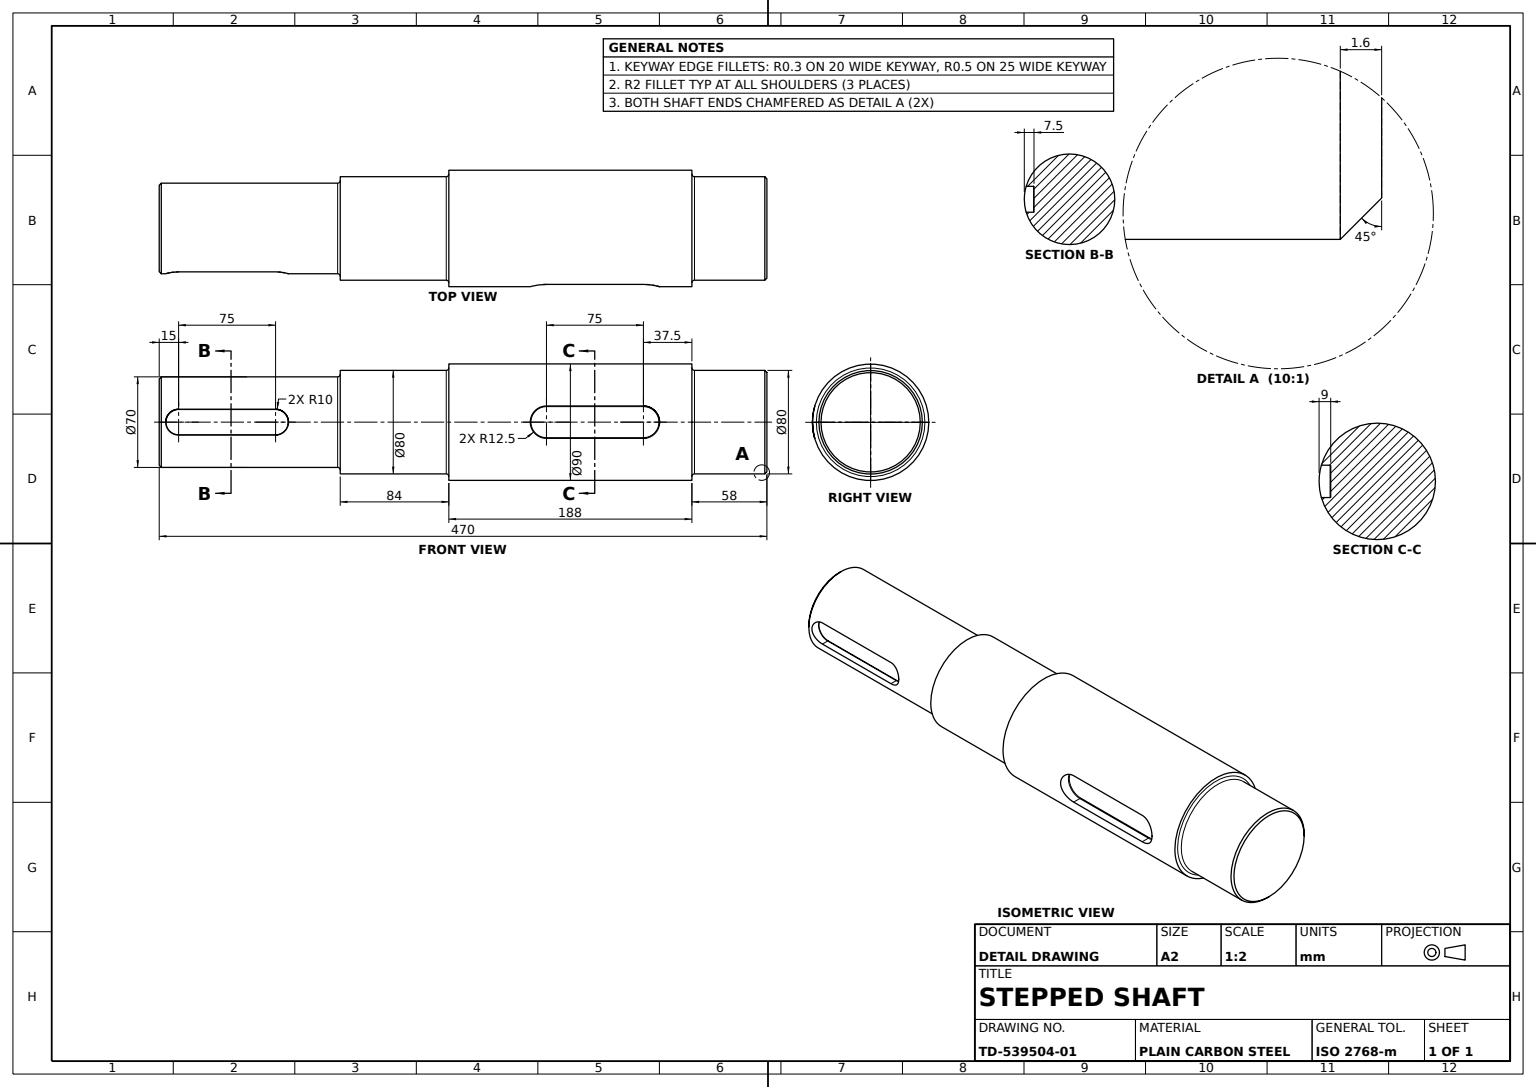
ISO-10303-21;
HEADER;
FILE_DESCRIPTION((''),'2;1');
FILE_NAME('','',(''),(''),'','','');
FILE_SCHEMA(('AUTOMOTIVE_DESIGN'));
ENDSEC;
DATA;
#1=APPLICATION_CONTEXT('');
#2=PRODUCT_CONTEXT('',#1,'mechanical');
#3=PRODUCT('','','',(#2));
#4=PRODUCT_DEFINITION_FORMATION('','',#3);
#5=PRODUCT_DEFINITION_CONTEXT('',#1,'design');
#6=PRODUCT_DEFINITION('','',#4,#5);
#7=PRODUCT_DEFINITION_SHAPE('','',#6);
#8=(LENGTH_UNIT()NAMED_UNIT(*)SI_UNIT(.MILLI.,.METRE.));
#9=(NAMED_UNIT(*)PLANE_ANGLE_UNIT()SI_UNIT($,.RADIAN.));
#10=(NAMED_UNIT(*)SI_UNIT($,.STERADIAN.)SOLID_ANGLE_UNIT());
#11=UNCERTAINTY_MEASURE_WITH_UNIT(LENGTH_MEASURE(1.E-05),#8,'distance_accuracy_value','');
#12=(GEOMETRIC_REPRESENTATION_CONTEXT(3)GLOBAL_UNCERTAINTY_ASSIGNED_CONTEXT((#11))GLOBAL_UNIT_ASSIGNED_CONTEXT((#8,#9,#10))REPRESENTATION_CONTEXT('',''));
#13=CARTESIAN_POINT('',(27.8,-10.,134.));
#14=VERTEX_POINT('',#13);
#15=CARTESIAN_POINT('',(27.5,-9.7,134.));
#16=VERTEX_POINT('',#15);
#17=CARTESIAN_POINT('',(27.8,-9.7,134.));
#18=DIRECTION('',(0.,0.,-1.));
#19=DIRECTION('',(-1.,0.,0.));
#20=AXIS2_PLACEMENT_3D('',#17,#18,#19);
#21=CIRCLE('',#20,0.3);
#22=EDGE_CURVE('',#14,#16,#21,.T.);
#23=ORIENTED_EDGE('',*,*,#22,.F.);
#24=CARTESIAN_POINT('',(27.8,0.,124.));
#25=VERTEX_POINT('',#24);
#26=CARTESIAN_POINT('',(27.8,0.,134.));
#27=AXIS2_PLACEMENT_3D('',#26,#19,#18);
#28=CIRCLE('',#27,10.);
#29=EDGE_CURVE('',#25,#14,#28,.T.);
#30=ORIENTED_EDGE('',*,*,#29,.F.);
#31=CARTESIAN_POINT('',(27.5,0.,124.3));
#32=VERTEX_POINT('',#31);
#33=CARTESIAN_POINT('',(27.8,0.,124.3));
#34=DIRECTION('',(0.,-1.,0.));
#35=AXIS2_PLACEMENT_3D('',#33,#34,#18);
#36=CIRCLE('',#35,0.3);
#37=EDGE_CURVE('',#32,#25,#36,.T.);
#38=ORIENTED_EDGE('',*,*,#37,.F.);
#39=CARTESIAN_POINT('',(27.5,0.,134.));
#40=DIRECTION('',(1.,0.,0.));
#41=AXIS2_PLACEMENT_3D('',#39,#40,#18);
#42=CIRCLE('',#41,9.7);
#43=EDGE_CURVE('',#16,#32,#42,.T.);
#44=ORIENTED_EDGE('',*,*,#43,.F.);
#45=EDGE_LOOP('',(#23,#30,#38,#44));
#46=FACE_OUTER_BOUND('',#45,.T.);
#47=AXIS2_PLACEMENT_3D('',#26,#40,#18);
#48=TOROIDAL_SURFACE('',#47,9.7,0.3);
#49=ADVANCED_FACE('',(#46),#48,.F.);
#50=CARTESIAN_POINT('',(40.,0.,84.));
#51=VERTEX_POINT('',#50);
#52=CARTESIAN_POINT('',(-40.,0.,84.));
#53=VERTEX_POINT('',#52);
#54=CARTESIAN_POINT('',(0.,0.,84.));
#55=DIRECTION('',(0.,0.,1.));
#56=AXIS2_PLACEMENT_3D('',#54,#55,#40);
#57=CIRCLE('',#56,40.);
#58=EDGE_CURVE('',#51,#53,#57,.T.);
#59=ORIENTED_EDGE('',*,*,#58,.T.);
#60=EDGE_CURVE('',#53,#51,#57,.T.);
#61=ORIENTED_EDGE('',*,*,#60,.T.);
#62=EDGE_LOOP('',(#59,#61));
#63=FACE_OUTER_BOUND('',#62,.T.);
#64=CARTESIAN_POINT('',(37.,0.,84.));
#65=VERTEX_POINT('',#64);
#66=CARTESIAN_POINT('',(-37.,0.,84.));
#67=VERTEX_POINT('',#66);
#68=AXIS2_PLACEMENT_3D('',#54,#18,#40);
#69=CIRCLE('',#68,37.);
#70=EDGE_CURVE('',#65,#67,#69,.T.);
#71=ORIENTED_EDGE('',*,*,#70,.T.);
#72=EDGE_CURVE('',#67,#65,#69,.T.);
#73=ORIENTED_EDGE('',*,*,#72,.T.);
#74=EDGE_LOOP('',(#71,#73));
#75=FACE_BOUND('',#74,.T.);
#76=CARTESIAN_POINT('',(0.,-35.,84.));
#77=AXIS2_PLACEMENT_3D('',#76,#55,#40);
#78=PLANE('',#77);
#79=ADVANCED_FACE('',(#63,#75),#78,.T.);
#80=CARTESIAN_POINT('',(36.,-12.,-75.5));
#81=VERTEX_POINT('',#80);
#82=CARTESIAN_POINT('',(36.5,-12.5,-75.5));
#83=VERTEX_POINT('',#82);
#84=CARTESIAN_POINT('',(36.5,-12.,-75.5));
#85=AXIS2_PLACEMENT_3D('',#84,#55,#40);
#86=CIRCLE('',#85,0.5);
#87=EDGE_CURVE('',#81,#83,#86,.T.);
#88=ORIENTED_EDGE('',*,*,#87,.F.);
#89=CARTESIAN_POINT('',(36.,12.,-75.5));
#90=VERTEX_POINT('',#89);
#91=CARTESIAN_POINT('',(36.,0.,-75.5));
#92=AXIS2_PLACEMENT_3D('',#91,#40,#18);
#93=CIRCLE('',#92,12.);
#94=EDGE_CURVE('',#90,#81,#93,.T.);
#95=ORIENTED_EDGE('',*,*,#94,.F.);
#96=CARTESIAN_POINT('',(36.5,12.5,-75.5));
#97=VERTEX_POINT('',#96);
#98=CARTESIAN_POINT('',(36.5,12.,-75.5));
#99=AXIS2_PLACEMENT_3D('',#98,#55,#40);
#100=CIRCLE('',#99,0.5);
#101=EDGE_CURVE('',#97,#90,#100,.T.);
#102=ORIENTED_EDGE('',*,*,#101,.F.);
#103=CARTESIAN_POINT('',(36.5,0.,-75.5));
#104=AXIS2_PLACEMENT_3D('',#103,#19,#18);
#105=CIRCLE('',#104,12.5);
#106=EDGE_CURVE('',#83,#97,#105,.T.);
#107=ORIENTED_EDGE('',*,*,#106,.F.);
#108=EDGE_LOOP('',(#88,#95,#102,#107));
#109=FACE_OUTER_BOUND('',#108,.T.);
#110=AXIS2_PLACEMENT_3D('',#103,#40,#18);
#111=TOROIDAL_SURFACE('',#110,12.,0.5);
#112=ADVANCED_FACE('',(#109),#111,.F.);
#113=CARTESIAN_POINT('',(40.,0.,-244.4));
#114=VERTEX_POINT('',#113);
#115=CARTESIAN_POINT('',(40.,0.,-190.));
#116=VERTEX_POINT('',#115);
#117=CARTESIAN_POINT('',(40.,0.,224.));
#118=VECTOR('',#55,1000.);
#119=LINE('',#117,#118);
#120=EDGE_CURVE('',#114,#116,#119,.T.);
#121=ORIENTED_EDGE('',*,*,#120,.T.);
#122=CARTESIAN_POINT('',(-40.,0.,-190.));
#123=VERTEX_POINT('',#122);
#124=CARTESIAN_POINT('',(0.,0.,-190.));
#125=AXIS2_PLACEMENT_3D('',#124,#18,#19);
#126=CIRCLE('',#125,40.);
#127=EDGE_CURVE('',#116,#123,#126,.T.);
#128=ORIENTED_EDGE('',*,*,#127,.T.);
#129=CARTESIAN_POINT('',(-40.,0.,-244.4));
#130=VERTEX_POINT('',#129);
#131=CARTESIAN_POINT('',(-40.,0.,224.));
#132=LINE('',#131,#118);
#133=EDGE_CURVE('',#130,#123,#132,.T.);
#134=ORIENTED_EDGE('',*,*,#133,.F.);
#135=CARTESIAN_POINT('',(0.,0.,-244.4));
#136=AXIS2_PLACEMENT_3D('',#135,#55,#19);
#137=CIRCLE('',#136,40.);
#138=EDGE_CURVE('',#130,#114,#137,.T.);
#139=ORIENTED_EDGE('',*,*,#138,.T.);
#140=EDGE_LOOP('',(#121,#128,#134,#139));
#141=FACE_OUTER_BOUND('',#140,.T.);
#142=CARTESIAN_POINT('',(0.,0.,224.));
#143=AXIS2_PLACEMENT_3D('',#142,#55,#40);
#144=CYLINDRICAL_SURFACE('',#143,40.);
#145=ADVANCED_FACE('',(#141),#144,.T.);
#146=CARTESIAN_POINT('',(27.5,9.7,209.));
#147=VERTEX_POINT('',#146);
#148=CARTESIAN_POINT('',(27.8,10.,209.));
#149=VERTEX_POINT('',#148);
#150=CARTESIAN_POINT('',(27.8,9.7,209.));
#151=AXIS2_PLACEMENT_3D('',#150,#18,#19);
#152=CIRCLE('',#151,0.3);
#153=EDGE_CURVE('',#147,#149,#152,.T.);
#154=ORIENTED_EDGE('',*,*,#153,.T.);
#155=CARTESIAN_POINT('',(27.8,-10.,209.));
#156=VERTEX_POINT('',#155);
#157=CARTESIAN_POINT('',(27.8,0.,209.));
#158=AXIS2_PLACEMENT_3D('',#157,#19,#18);
#159=CIRCLE('',#158,10.);
#160=EDGE_CURVE('',#156,#149,#159,.T.);
#161=ORIENTED_EDGE('',*,*,#160,.F.);
#162=CARTESIAN_POINT('',(27.5,-9.7,209.));
#163=VERTEX_POINT('',#162);
#164=CARTESIAN_POINT('',(27.8,-9.7,209.));
#165=AXIS2_PLACEMENT_3D('',#164,#55,#40);
#166=CIRCLE('',#165,0.3);
#167=EDGE_CURVE('',#163,#156,#166,.T.);
#168=ORIENTED_EDGE('',*,*,#167,.F.);
#169=CARTESIAN_POINT('',(27.5,0.,209.));
#170=AXIS2_PLACEMENT_3D('',#169,#40,#18);
#171=CIRCLE('',#170,9.7);
#172=EDGE_CURVE('',#147,#163,#171,.T.);
#173=ORIENTED_EDGE('',*,*,#172,.F.);
#174=EDGE_LOOP('',(#154,#161,#168,#173));
#175=FACE_OUTER_BOUND('',#174,.T.);
#176=AXIS2_PLACEMENT_3D('',#157,#40,#18);
#177=TOROIDAL_SURFACE('',#176,9.7,0.3);
#178=ADVANCED_FACE('',(#175),#177,.F.);
#179=CARTESIAN_POINT('',(38.4,0.,-246.));
#180=VERTEX_POINT('',#179);
#181=CARTESIAN_POINT('',(-38.4,0.,-246.));
#182=VERTEX_POINT('',#181);
#183=CARTESIAN_POINT('',(0.,0.,-246.));
#184=AXIS2_PLACEMENT_3D('',#183,#18,#19);
#185=CIRCLE('',#184,38.4);
#186=EDGE_CURVE('',#180,#182,#185,.T.);
#187=ORIENTED_EDGE('',*,*,#186,.F.);
#188=DIRECTION('',(0.707106781,0.,0.707106781));
#189=VECTOR('',#188,1000.);
#190=LINE('',#113,#189);
#191=EDGE_CURVE('',#180,#114,#190,.T.);
#192=ORIENTED_EDGE('',*,*,#191,.T.);
#193=ORIENTED_EDGE('',*,*,#138,.F.);
#194=DIRECTION('',(-0.707106781,0.,0.707106781));
#195=VECTOR('',#194,1000.);
#196=LINE('',#129,#195);
#197=EDGE_CURVE('',#182,#130,#196,.T.);
#198=ORIENTED_EDGE('',*,*,#197,.F.);
#199=EDGE_LOOP('',(#187,#192,#193,#198));
#200=FACE_OUTER_BOUND('',#199,.T.);
#201=AXIS2_PLACEMENT_3D('',#135,#55,#40);
#202=CONICAL_SURFACE('',#201,40.,0.785398163);
#203=ADVANCED_FACE('',(#200),#202,.T.);
#204=CARTESIAN_POINT('',(42.,0.,0.));
#205=VERTEX_POINT('',#204);
#206=CARTESIAN_POINT('',(-42.,0.,0.));
#207=VERTEX_POINT('',#206);
#208=CARTESIAN_POINT('',(0.,0.,0.));
#209=AXIS2_PLACEMENT_3D('',#208,#18,#40);
#210=CIRCLE('',#209,42.);
#211=EDGE_CURVE('',#205,#207,#210,.T.);
#212=ORIENTED_EDGE('',*,*,#211,.F.);
#213=CARTESIAN_POINT('',(40.,0.,2.));
#214=VERTEX_POINT('',#213);
#215=CARTESIAN_POINT('',(42.,0.,2.));
#216=AXIS2_PLACEMENT_3D('',#215,#34,#18);
#217=CIRCLE('',#216,2.);
#218=EDGE_CURVE('',#214,#205,#217,.T.);
#219=ORIENTED_EDGE('',*,*,#218,.F.);
#220=CARTESIAN_POINT('',(-40.,0.,2.));
#221=VERTEX_POINT('',#220);
#222=CARTESIAN_POINT('',(0.,0.,2.));
#223=AXIS2_PLACEMENT_3D('',#222,#55,#40);
#224=CIRCLE('',#223,40.);
#225=EDGE_CURVE('',#221,#214,#224,.T.);
#226=ORIENTED_EDGE('',*,*,#225,.F.);
#227=CARTESIAN_POINT('',(-42.,0.,2.));
#228=DIRECTION('',(0.,1.,0.));
#229=AXIS2_PLACEMENT_3D('',#227,#228,#19);
#230=CIRCLE('',#229,2.);
#231=EDGE_CURVE('',#221,#207,#230,.T.);
#232=ORIENTED_EDGE('',*,*,#231,.T.);
#233=EDGE_LOOP('',(#212,#219,#226,#232));
#234=FACE_OUTER_BOUND('',#233,.T.);
#235=TOROIDAL_SURFACE('',#223,42.,2.);
#236=ADVANCED_FACE('',(#234),#235,.F.);
#237=CARTESIAN_POINT('',(43.229041,12.5,-75.5));
#238=VERTEX_POINT('',#237);
#239=CARTESIAN_POINT('',(45.,0.,-63.));
#240=VERTEX_POINT('',#239);
#241=CARTESIAN_POINT('',(43.229041,12.5,-74.669444));
#242=CARTESIAN_POINT('',(43.252973,12.418052,-73.853634));
#243=CARTESIAN_POINT('',(43.320977,12.177845,-72.650927));
#244=CARTESIAN_POINT('',(43.348996,12.07808,-72.253551));
#245=CARTESIAN_POINT('',(43.415084,11.838325,-71.465957));
#246=CARTESIAN_POINT('',(43.453231,11.697998,-71.075695));
#247=CARTESIAN_POINT('',(43.57844,11.226107,-69.941668));
#248=CARTESIAN_POINT('',(43.67694,10.841696,-69.225197));
#249=CARTESIAN_POINT('',(43.838424,10.161049,-68.20826));
#250=CARTESIAN_POINT('',(43.894862,9.915236,-67.877304));
#251=CARTESIAN_POINT('',(44.00903,9.395534,-67.245223));
#252=CARTESIAN_POINT('',(44.066707,9.122003,-66.944091));
#253=CARTESIAN_POINT('',(44.239067,8.261203,-66.084024));
#254=CARTESIAN_POINT('',(44.353104,7.634144,-65.567968));
#255=CARTESIAN_POINT('',(44.513291,6.60957,-64.882447));
#256=CARTESIAN_POINT('',(44.564301,6.257358,-64.671259));
#257=CARTESIAN_POINT('',(44.659332,5.538545,-64.286585));
#258=CARTESIAN_POINT('',(44.703518,5.170919,-64.112408));
#259=CARTESIAN_POINT('',(44.784077,4.419198,-63.800157));
#260=CARTESIAN_POINT('',(44.820454,4.035104,-63.66208));
#261=CARTESIAN_POINT('',(44.884218,3.24994,-63.422901));
#262=CARTESIAN_POINT('',(44.911703,2.846524,-63.321452));
#263=CARTESIAN_POINT('',(44.977592,1.63437,-63.079944));
#264=CARTESIAN_POINT('',(45.,0.820192,-63.));
#265=B_SPLINE_CURVE_WITH_KNOTS('',3,(#237,#241,#242,#243,#244,#245,#246,#247,#248,#249,#250,#251,#252,#253,#254,#255,#256,#257,#258,#259,#260,#261,#262,#263,#264,#239),.UNSPECIFIED.,.F.,.F.,(4,2,2,2,2,2,2,2,2,2,2,2,4),(0.,0.002455301,0.003682952,0.004910602,0.007365903,0.008593554,0.009821204,0.012276505,0.013504156,0.014731806,0.015959457,0.017187107,0.019642408),.UNSPECIFIED.);
#266=EDGE_CURVE('',#238,#240,#265,.T.);
#267=ORIENTED_EDGE('',*,*,#266,.T.);
#268=CARTESIAN_POINT('',(43.229041,-12.5,-75.5));
#269=VERTEX_POINT('',#268);
#270=CARTESIAN_POINT('',(45.,-0.819211,-63.));
#271=CARTESIAN_POINT('',(44.976869,-1.651428,-63.082566));
#272=CARTESIAN_POINT('',(44.889211,-3.256491,-63.40392));
#273=CARTESIAN_POINT('',(44.825036,-4.03713,-63.641391));
#274=CARTESIAN_POINT('',(44.703051,-5.175208,-64.114221));
#275=CARTESIAN_POINT('',(44.65811,-5.548408,-64.291443));
#276=CARTESIAN_POINT('',(44.562841,-6.267761,-64.677258));
#277=CARTESIAN_POINT('',(44.512297,-6.61603,-64.886672));
#278=CARTESIAN_POINT('',(44.406845,-7.290307,-65.338011));
#279=CARTESIAN_POINT('',(44.351934,-7.616315,-65.579937));
#280=CARTESIAN_POINT('',(44.239196,-8.245959,-66.096805));
#281=CARTESIAN_POINT('',(44.181054,-8.551092,-66.373362));
#282=CARTESIAN_POINT('',(44.00756,-9.417079,-67.23953));
#283=CARTESIAN_POINT('',(43.892946,-9.931025,-67.865591));
#284=CARTESIAN_POINT('',(43.732114,-10.60925,-68.877412));
#285=CARTESIAN_POINT('',(43.68035,-10.819759,-69.226896));
#286=CARTESIAN_POINT('',(43.5822,-11.208569,-69.951397));
#287=CARTESIAN_POINT('',(43.536404,-11.384542,-70.322313));
#288=CARTESIAN_POINT('',(43.411743,-11.854347,-71.451622));
#289=CARTESIAN_POINT('',(43.345077,-12.092668,-72.230171));
#290=CARTESIAN_POINT('',(43.276334,-12.335559,-73.437819));
#291=CARTESIAN_POINT('',(43.258611,-12.397354,-73.848719));
#292=CARTESIAN_POINT('',(43.235012,-12.479404,-74.671989));
#293=CARTESIAN_POINT('',(43.229041,-12.5,-75.0852));
#294=B_SPLINE_CURVE_WITH_KNOTS('',3,(#239,#270,#271,#272,#273,#274,#275,#276,#277,#278,#279,#280,#281,#282,#283,#284,#285,#286,#287,#288,#289,#290,#291,#292,#293,#268),.UNSPECIFIED.,.F.,.F.,(4,2,2,2,2,2,2,2,2,2,2,2,4),(0.019642408,0.022094774,0.024547139,0.025773322,0.026999505,0.028225688,0.02945187,0.031904236,0.033130419,0.034356602,0.036808967,0.03803515,0.039261333),.UNSPECIFIED.);
#295=EDGE_CURVE('',#240,#269,#294,.T.);
#296=ORIENTED_EDGE('',*,*,#295,.T.);
#297=CARTESIAN_POINT('',(36.,-12.5,-75.5));
#298=VECTOR('',#40,1000.);
#299=LINE('',#297,#298);
#300=EDGE_CURVE('',#83,#269,#299,.T.);
#301=ORIENTED_EDGE('',*,*,#300,.F.);
#302=ORIENTED_EDGE('',*,*,#106,.T.);
#303=CARTESIAN_POINT('',(36.,12.5,-75.5));
#304=LINE('',#303,#298);
#305=EDGE_CURVE('',#97,#238,#304,.T.);
#306=ORIENTED_EDGE('',*,*,#305,.T.);
#307=EDGE_LOOP('',(#267,#296,#301,#302,#306));
#308=FACE_OUTER_BOUND('',#307,.T.);
#309=CYLINDRICAL_SURFACE('',#92,12.5);
#310=ADVANCED_FACE('',(#308),#309,.F.);
#311=CARTESIAN_POINT('',(43.229041,-12.5,-150.5));
#312=VERTEX_POINT('',#311);
#313=CARTESIAN_POINT('',(45.,0.,-163.));
#314=VERTEX_POINT('',#313);
#315=CARTESIAN_POINT('',(43.229041,-12.5,-151.330556));
#316=CARTESIAN_POINT('',(43.252973,-12.418052,-152.146366));
#317=CARTESIAN_POINT('',(43.320977,-12.177845,-153.349073));
#318=CARTESIAN_POINT('',(43.348996,-12.07808,-153.746449));
#319=CARTESIAN_POINT('',(43.415084,-11.838325,-154.534043));
#320=CARTESIAN_POINT('',(43.453231,-11.697998,-154.924305));
#321=CARTESIAN_POINT('',(43.57844,-11.226107,-156.058332));
#322=CARTESIAN_POINT('',(43.67694,-10.841696,-156.774803));
#323=CARTESIAN_POINT('',(43.838424,-10.161049,-157.79174));
#324=CARTESIAN_POINT('',(43.894862,-9.915236,-158.122696));
#325=CARTESIAN_POINT('',(44.00903,-9.395534,-158.754777));
#326=CARTESIAN_POINT('',(44.066707,-9.122003,-159.055909));
#327=CARTESIAN_POINT('',(44.239067,-8.261203,-159.915976));
#328=CARTESIAN_POINT('',(44.353104,-7.634144,-160.432032));
#329=CARTESIAN_POINT('',(44.513291,-6.60957,-161.117553));
#330=CARTESIAN_POINT('',(44.564301,-6.257358,-161.328741));
#331=CARTESIAN_POINT('',(44.659332,-5.538545,-161.713415));
#332=CARTESIAN_POINT('',(44.703518,-5.170919,-161.887592));
#333=CARTESIAN_POINT('',(44.784077,-4.419198,-162.199843));
#334=CARTESIAN_POINT('',(44.820454,-4.035104,-162.33792));
#335=CARTESIAN_POINT('',(44.884218,-3.24994,-162.577099));
#336=CARTESIAN_POINT('',(44.911703,-2.846524,-162.678548));
#337=CARTESIAN_POINT('',(44.977592,-1.63437,-162.920056));
#338=CARTESIAN_POINT('',(45.,-0.820192,-163.));
#339=B_SPLINE_CURVE_WITH_KNOTS('',3,(#311,#315,#316,#317,#318,#319,#320,#321,#322,#323,#324,#325,#326,#327,#328,#329,#330,#331,#332,#333,#334,#335,#336,#337,#338,#313),.UNSPECIFIED.,.F.,.F.,(4,2,2,2,2,2,2,2,2,2,2,2,4),(0.,0.002455301,0.003682952,0.004910602,0.007365903,0.008593554,0.009821204,0.012276505,0.013504156,0.014731806,0.015959457,0.017187107,0.019642408),.UNSPECIFIED.);
#340=EDGE_CURVE('',#312,#314,#339,.T.);
#341=ORIENTED_EDGE('',*,*,#340,.T.);
#342=CARTESIAN_POINT('',(36.5,0.,-163.));
#343=VERTEX_POINT('',#342);
#344=CARTESIAN_POINT('',(36.,0.,-163.));
#345=LINE('',#344,#298);
#346=EDGE_CURVE('',#343,#314,#345,.T.);
#347=ORIENTED_EDGE('',*,*,#346,.F.);
#348=CARTESIAN_POINT('',(36.5,-12.5,-150.5));
#349=VERTEX_POINT('',#348);
#350=CARTESIAN_POINT('',(36.5,0.,-150.5));
#351=AXIS2_PLACEMENT_3D('',#350,#19,#18);
#352=CIRCLE('',#351,12.5);
#353=EDGE_CURVE('',#343,#349,#352,.T.);
#354=ORIENTED_EDGE('',*,*,#353,.T.);
#355=CARTESIAN_POINT('',(36.,-12.5,-150.5));
#356=LINE('',#355,#298);
#357=EDGE_CURVE('',#349,#312,#356,.T.);
#358=ORIENTED_EDGE('',*,*,#357,.T.);
#359=EDGE_LOOP('',(#341,#347,#354,#358));
#360=FACE_OUTER_BOUND('',#359,.T.);
#361=CARTESIAN_POINT('',(36.,0.,-150.5));
#362=AXIS2_PLACEMENT_3D('',#361,#40,#18);
#363=CYLINDRICAL_SURFACE('',#362,12.5);
#364=ADVANCED_FACE('',(#360),#363,.F.);
#365=CARTESIAN_POINT('',(33.54102,-10.,209.));
#366=VERTEX_POINT('',#365);
#367=CARTESIAN_POINT('',(33.54102,-10.,134.));
#368=VERTEX_POINT('',#367);
#369=CARTESIAN_POINT('',(33.54102,-10.,224.));
#370=VECTOR('',#18,1000.);
#371=LINE('',#369,#370);
#372=EDGE_CURVE('',#366,#368,#371,.T.);
#373=ORIENTED_EDGE('',*,*,#372,.T.);
#374=CARTESIAN_POINT('',(27.5,-10.,134.));
#375=LINE('',#374,#298);
#376=EDGE_CURVE('',#14,#368,#375,.T.);
#377=ORIENTED_EDGE('',*,*,#376,.F.);
#378=LINE('',#155,#118);
#379=EDGE_CURVE('',#14,#156,#378,.T.);
#380=ORIENTED_EDGE('',*,*,#379,.T.);
#381=CARTESIAN_POINT('',(27.5,-10.,209.));
#382=LINE('',#381,#298);
#383=EDGE_CURVE('',#156,#366,#382,.T.);
#384=ORIENTED_EDGE('',*,*,#383,.T.);
#385=EDGE_LOOP('',(#373,#377,#380,#384));
#386=FACE_OUTER_BOUND('',#385,.T.);
#387=AXIS2_PLACEMENT_3D('',#381,#34,#18);
#388=PLANE('',#387);
#389=ADVANCED_FACE('',(#386),#388,.F.);
#390=ORIENTED_EDGE('',*,*,#70,.F.);
#391=CARTESIAN_POINT('',(35.,0.,86.));
#392=VERTEX_POINT('',#391);
#393=CARTESIAN_POINT('',(37.,0.,86.));
#394=AXIS2_PLACEMENT_3D('',#393,#34,#18);
#395=CIRCLE('',#394,2.);
#396=EDGE_CURVE('',#392,#65,#395,.T.);
#397=ORIENTED_EDGE('',*,*,#396,.F.);
#398=CARTESIAN_POINT('',(-35.,0.,86.));
#399=VERTEX_POINT('',#398);
#400=CARTESIAN_POINT('',(0.,0.,86.));
#401=AXIS2_PLACEMENT_3D('',#400,#55,#40);
#402=CIRCLE('',#401,35.);
#403=EDGE_CURVE('',#399,#392,#402,.T.);
#404=ORIENTED_EDGE('',*,*,#403,.F.);
#405=CARTESIAN_POINT('',(-37.,0.,86.));
#406=AXIS2_PLACEMENT_3D('',#405,#228,#19);
#407=CIRCLE('',#406,2.);
#408=EDGE_CURVE('',#399,#67,#407,.T.);
#409=ORIENTED_EDGE('',*,*,#408,.T.);
#410=EDGE_LOOP('',(#390,#397,#404,#409));
#411=FACE_OUTER_BOUND('',#410,.T.);
#412=TOROIDAL_SURFACE('',#401,37.,2.);
#413=ADVANCED_FACE('',(#411),#412,.F.);
#414=CARTESIAN_POINT('',(27.8,10.,134.));
#415=VERTEX_POINT('',#414);
#416=CARTESIAN_POINT('',(33.54102,10.,134.));
#417=VERTEX_POINT('',#416);
#418=CARTESIAN_POINT('',(27.5,10.,134.));
#419=LINE('',#418,#298);
#420=EDGE_CURVE('',#415,#417,#419,.T.);
#421=ORIENTED_EDGE('',*,*,#420,.F.);
#422=EDGE_CURVE('',#415,#25,#28,.T.);
#423=ORIENTED_EDGE('',*,*,#422,.T.);
#424=CARTESIAN_POINT('',(35.,0.,124.));
#425=VERTEX_POINT('',#424);
#426=CARTESIAN_POINT('',(27.5,0.,124.));
#427=LINE('',#426,#298);
#428=EDGE_CURVE('',#25,#425,#427,.T.);
#429=ORIENTED_EDGE('',*,*,#428,.T.);
#430=CARTESIAN_POINT('',(35.,0.65559,124.));
#431=CARTESIAN_POINT('',(34.980953,1.321562,124.066103));
#432=CARTESIAN_POINT('',(34.908789,2.605779,124.323288));
#433=CARTESIAN_POINT('',(34.855955,3.230397,124.513337));
#434=CARTESIAN_POINT('',(34.755502,4.141058,124.891778));
#435=CARTESIAN_POINT('',(34.718515,4.439483,125.033532));
#436=CARTESIAN_POINT('',(34.640094,5.014794,125.342148));
#437=CARTESIAN_POINT('',(34.598485,5.29334,125.509661));
#438=CARTESIAN_POINT('',(34.51166,5.83266,125.870709));
#439=CARTESIAN_POINT('',(34.466442,6.093434,126.064243));
#440=CARTESIAN_POINT('',(34.373589,6.597118,126.477752));
#441=CARTESIAN_POINT('',(34.325699,6.841193,126.698998));
#442=CARTESIAN_POINT('',(34.182859,7.533541,127.391524));
#443=CARTESIAN_POINT('',(34.088449,7.944574,127.892159));
#444=CARTESIAN_POINT('',(33.911714,8.668003,128.971312));
#445=CARTESIAN_POINT('',(33.828827,8.982089,129.556196));
#446=CARTESIAN_POINT('',(33.691792,9.483174,130.760443));
#447=CARTESIAN_POINT('',(33.636786,9.673926,131.383295));
#448=CARTESIAN_POINT('',(33.580049,9.868378,132.349817));
#449=CARTESIAN_POINT('',(33.565421,9.917847,132.67869));
#450=CARTESIAN_POINT('',(33.545948,9.983513,133.337411));
#451=CARTESIAN_POINT('',(33.54102,10.,133.668056));
#452=B_SPLINE_CURVE_WITH_KNOTS('',3,(#424,#430,#431,#432,#433,#434,#435,#436,#437,#438,#439,#440,#441,#442,#443,#444,#445,#446,#447,#448,#449,#450,#451,#416),.UNSPECIFIED.,.F.,.F.,(4,2,2,2,2,2,2,2,2,2,2,4),(0.015718611,0.01768105,0.019643488,0.020624708,0.021605927,0.022587146,0.023568366,0.025530805,0.027493243,0.029455682,0.030436901,0.031418121),.UNSPECIFIED.);
#453=EDGE_CURVE('',#425,#417,#452,.T.);
#454=ORIENTED_EDGE('',*,*,#453,.T.);
#455=EDGE_LOOP('',(#421,#423,#429,#454));
#456=FACE_OUTER_BOUND('',#455,.T.);
#457=CYLINDRICAL_SURFACE('',#41,10.);
#458=ADVANCED_FACE('',(#456),#457,.F.);
#459=LINE('',#414,#370);
#460=EDGE_CURVE('',#149,#415,#459,.T.);
#461=ORIENTED_EDGE('',*,*,#460,.T.);
#462=ORIENTED_EDGE('',*,*,#420,.T.);
#463=CARTESIAN_POINT('',(33.54102,10.,209.));
#464=VERTEX_POINT('',#463);
#465=CARTESIAN_POINT('',(33.54102,10.,224.));
#466=LINE('',#465,#370);
#467=EDGE_CURVE('',#464,#417,#466,.T.);
#468=ORIENTED_EDGE('',*,*,#467,.F.);
#469=CARTESIAN_POINT('',(27.5,10.,209.));
#470=LINE('',#469,#298);
#471=EDGE_CURVE('',#149,#464,#470,.T.);
#472=ORIENTED_EDGE('',*,*,#471,.F.);
#473=EDGE_LOOP('',(#461,#462,#468,#472));
#474=FACE_OUTER_BOUND('',#473,.T.);
#475=AXIS2_PLACEMENT_3D('',#469,#34,#18);
#476=PLANE('',#475);
#477=ADVANCED_FACE('',(#474),#476,.T.);
#478=CARTESIAN_POINT('',(42.,0.,-188.));
#479=VERTEX_POINT('',#478);
#480=CARTESIAN_POINT('',(42.,0.,-190.));
#481=AXIS2_PLACEMENT_3D('',#480,#228,#19);
#482=CIRCLE('',#481,2.);
#483=EDGE_CURVE('',#116,#479,#482,.T.);
#484=ORIENTED_EDGE('',*,*,#483,.T.);
#485=CARTESIAN_POINT('',(-42.,0.,-188.));
#486=VERTEX_POINT('',#485);
#487=CARTESIAN_POINT('',(0.,0.,-188.));
#488=AXIS2_PLACEMENT_3D('',#487,#55,#19);
#489=CIRCLE('',#488,42.);
#490=EDGE_CURVE('',#486,#479,#489,.T.);
#491=ORIENTED_EDGE('',*,*,#490,.F.);
#492=CARTESIAN_POINT('',(-42.,0.,-190.));
#493=AXIS2_PLACEMENT_3D('',#492,#34,#18);
#494=CIRCLE('',#493,2.);
#495=EDGE_CURVE('',#123,#486,#494,.T.);
#496=ORIENTED_EDGE('',*,*,#495,.F.);
#497=ORIENTED_EDGE('',*,*,#127,.F.);
#498=EDGE_LOOP('',(#484,#491,#496,#497));
#499=FACE_OUTER_BOUND('',#498,.T.);
#500=TOROIDAL_SURFACE('',#125,42.,2.);
#501=ADVANCED_FACE('',(#499),#500,.F.);
#502=ORIENTED_EDGE('',*,*,#460,.F.);
#503=ORIENTED_EDGE('',*,*,#153,.F.);
#504=CARTESIAN_POINT('',(27.5,9.7,134.));
#505=VERTEX_POINT('',#504);
#506=LINE('',#146,#118);
#507=EDGE_CURVE('',#505,#147,#506,.T.);
#508=ORIENTED_EDGE('',*,*,#507,.F.);
#509=CARTESIAN_POINT('',(27.8,9.7,134.));
#510=AXIS2_PLACEMENT_3D('',#509,#55,#40);
#511=CIRCLE('',#510,0.3);
#512=EDGE_CURVE('',#415,#505,#511,.T.);
#513=ORIENTED_EDGE('',*,*,#512,.F.);
#514=EDGE_LOOP('',(#502,#503,#508,#513));
#515=FACE_OUTER_BOUND('',#514,.T.);
#516=AXIS2_PLACEMENT_3D('',#150,#55,#34);
#517=CYLINDRICAL_SURFACE('',#516,0.3);
#518=ADVANCED_FACE('',(#515),#517,.F.);
#519=ORIENTED_EDGE('',*,*,#172,.T.);
#520=LINE('',#162,#370);
#521=EDGE_CURVE('',#163,#16,#520,.T.);
#522=ORIENTED_EDGE('',*,*,#521,.T.);
#523=ORIENTED_EDGE('',*,*,#43,.T.);
#524=EDGE_CURVE('',#32,#505,#42,.T.);
#525=ORIENTED_EDGE('',*,*,#524,.T.);
#526=ORIENTED_EDGE('',*,*,#507,.T.);
#527=EDGE_LOOP('',(#519,#522,#523,#525,#526));
#528=FACE_OUTER_BOUND('',#527,.T.);
#529=PLANE('',#170);
#530=ADVANCED_FACE('',(#528),#529,.T.);
#531=CARTESIAN_POINT('',(35.,0.,222.4));
#532=VERTEX_POINT('',#531);
#533=CARTESIAN_POINT('',(-35.,0.,222.4));
#534=VERTEX_POINT('',#533);
#535=CARTESIAN_POINT('',(0.,0.,222.4));
#536=AXIS2_PLACEMENT_3D('',#535,#18,#40);
#537=CIRCLE('',#536,35.);
#538=EDGE_CURVE('',#532,#534,#537,.T.);
#539=ORIENTED_EDGE('',*,*,#538,.T.);
#540=CARTESIAN_POINT('',(-35.,0.,224.));
#541=LINE('',#540,#118);
#542=EDGE_CURVE('',#399,#534,#541,.T.);
#543=ORIENTED_EDGE('',*,*,#542,.F.);
#544=ORIENTED_EDGE('',*,*,#403,.T.);
#545=CARTESIAN_POINT('',(35.,0.,224.));
#546=LINE('',#545,#118);
#547=EDGE_CURVE('',#392,#425,#546,.T.);
#548=ORIENTED_EDGE('',*,*,#547,.T.);
#549=CARTESIAN_POINT('',(33.54102,-10.,133.33534));
#550=CARTESIAN_POINT('',(33.560774,-9.9344,132.682524));
#551=CARTESIAN_POINT('',(33.616887,-9.742143,131.720163));
#552=CARTESIAN_POINT('',(33.640006,-9.662295,131.402206));
#553=CARTESIAN_POINT('',(33.694528,-9.470414,130.772037));
#554=CARTESIAN_POINT('',(33.725991,-9.358129,130.459845));
#555=CARTESIAN_POINT('',(33.829239,-8.980571,129.552705));
#556=CARTESIAN_POINT('',(33.910442,-8.673036,128.979612));
#557=CARTESIAN_POINT('',(34.04353,-8.12853,128.16618));
#558=CARTESIAN_POINT('',(34.090037,-7.931885,127.901455));
#559=CARTESIAN_POINT('',(34.184074,-7.516282,127.39602));
#560=CARTESIAN_POINT('',(34.231577,-7.297537,127.155208));
#561=CARTESIAN_POINT('',(34.373525,-6.609114,126.46737));
#562=CARTESIAN_POINT('',(34.46743,-6.107586,126.054583));
#563=CARTESIAN_POINT('',(34.643306,-5.014746,125.323331));
#564=CARTESIAN_POINT('',(34.722752,-4.438075,125.01515));
#565=CARTESIAN_POINT('',(34.822233,-3.536046,124.640385));
#566=CARTESIAN_POINT('',(34.852181,-3.22875,124.529889));
#567=CARTESIAN_POINT('',(34.904681,-2.600495,124.338465));
#568=CARTESIAN_POINT('',(34.92731,-2.277677,124.257267));
#569=CARTESIAN_POINT('',(34.981549,-1.307872,124.064001));
#570=CARTESIAN_POINT('',(35.,-0.656388,124.));
#571=B_SPLINE_CURVE_WITH_KNOTS('',3,(#367,#549,#550,#551,#552,#553,#554,#555,#556,#557,#558,#559,#560,#561,#562,#563,#564,#565,#566,#567,#568,#569,#570,#424),.UNSPECIFIED.,.F.,.F.,(4,2,2,2,2,2,2,2,2,2,2,4),(0.,0.001964826,0.00294724,0.003929653,0.005894479,0.006876892,0.007859305,0.009824132,0.011788958,0.012771371,0.013753784,0.015718611),.UNSPECIFIED.);
#572=EDGE_CURVE('',#368,#425,#571,.T.);
#573=ORIENTED_EDGE('',*,*,#572,.F.);
#574=ORIENTED_EDGE('',*,*,#372,.F.);
#575=CARTESIAN_POINT('',(35.,0.,219.));
#576=VERTEX_POINT('',#575);
#577=CARTESIAN_POINT('',(35.,-0.65559,219.));
#578=CARTESIAN_POINT('',(34.980953,-1.321562,218.933897));
#579=CARTESIAN_POINT('',(34.908789,-2.605779,218.676712));
#580=CARTESIAN_POINT('',(34.855955,-3.230397,218.486663));
#581=CARTESIAN_POINT('',(34.755502,-4.141058,218.108222));
#582=CARTESIAN_POINT('',(34.718515,-4.439483,217.966468));
#583=CARTESIAN_POINT('',(34.640094,-5.014794,217.657852));
#584=CARTESIAN_POINT('',(34.598485,-5.29334,217.490339));
#585=CARTESIAN_POINT('',(34.51166,-5.83266,217.129291));
#586=CARTESIAN_POINT('',(34.466442,-6.093434,216.935757));
#587=CARTESIAN_POINT('',(34.373589,-6.597118,216.522248));
#588=CARTESIAN_POINT('',(34.325699,-6.841193,216.301002));
#589=CARTESIAN_POINT('',(34.182859,-7.533541,215.608476));
#590=CARTESIAN_POINT('',(34.088449,-7.944574,215.107841));
#591=CARTESIAN_POINT('',(33.911714,-8.668003,214.028688));
#592=CARTESIAN_POINT('',(33.828827,-8.982089,213.443804));
#593=CARTESIAN_POINT('',(33.691792,-9.483174,212.239557));
#594=CARTESIAN_POINT('',(33.636786,-9.673926,211.616705));
#595=CARTESIAN_POINT('',(33.580049,-9.868378,210.650183));
#596=CARTESIAN_POINT('',(33.565421,-9.917847,210.32131));
#597=CARTESIAN_POINT('',(33.545948,-9.983513,209.662589));
#598=CARTESIAN_POINT('',(33.54102,-10.,209.331944));
#599=B_SPLINE_CURVE_WITH_KNOTS('',3,(#575,#577,#578,#579,#580,#581,#582,#583,#584,#585,#586,#587,#588,#589,#590,#591,#592,#593,#594,#595,#596,#597,#598,#365),.UNSPECIFIED.,.F.,.F.,(4,2,2,2,2,2,2,2,2,2,2,4),(0.015718611,0.01768105,0.019643488,0.020624708,0.021605927,0.022587146,0.023568366,0.025530805,0.027493243,0.029455682,0.030436901,0.031418121),.UNSPECIFIED.);
#600=EDGE_CURVE('',#576,#366,#599,.T.);
#601=ORIENTED_EDGE('',*,*,#600,.F.);
#602=EDGE_CURVE('',#576,#532,#546,.T.);
#603=ORIENTED_EDGE('',*,*,#602,.T.);
#604=EDGE_LOOP('',(#539,#543,#544,#548,#573,#574,#601,#603));
#605=FACE_OUTER_BOUND('',#604,.T.);
#606=CYLINDRICAL_SURFACE('',#143,35.);
#607=ADVANCED_FACE('',(#605),#606,.T.);
#608=CARTESIAN_POINT('',(45.,0.,-188.));
#609=VERTEX_POINT('',#608);
#610=CARTESIAN_POINT('',(45.,0.,224.));
#611=LINE('',#610,#118);
#612=EDGE_CURVE('',#609,#314,#611,.T.);
#613=ORIENTED_EDGE('',*,*,#612,.F.);
#614=CARTESIAN_POINT('',(-45.,0.,-188.));
#615=VERTEX_POINT('',#614);
#616=AXIS2_PLACEMENT_3D('',#487,#55,#40);
#617=CIRCLE('',#616,45.);
#618=EDGE_CURVE('',#609,#615,#617,.T.);
#619=ORIENTED_EDGE('',*,*,#618,.T.);
#620=CARTESIAN_POINT('',(-45.,0.,0.));
#621=VERTEX_POINT('',#620);
#622=CARTESIAN_POINT('',(-45.,0.,224.));
#623=LINE('',#622,#118);
#624=EDGE_CURVE('',#615,#621,#623,.T.);
#625=ORIENTED_EDGE('',*,*,#624,.T.);
#626=CARTESIAN_POINT('',(45.,0.,0.));
#627=VERTEX_POINT('',#626);
#628=AXIS2_PLACEMENT_3D('',#208,#55,#40);
#629=CIRCLE('',#628,45.);
#630=EDGE_CURVE('',#627,#621,#629,.T.);
#631=ORIENTED_EDGE('',*,*,#630,.F.);
#632=EDGE_CURVE('',#240,#627,#611,.T.);
#633=ORIENTED_EDGE('',*,*,#632,.F.);
#634=ORIENTED_EDGE('',*,*,#266,.F.);
#635=CARTESIAN_POINT('',(43.229041,12.5,-150.5));
#636=VERTEX_POINT('',#635);
#637=CARTESIAN_POINT('',(43.229041,12.5,224.));
#638=LINE('',#637,#370);
#639=EDGE_CURVE('',#238,#636,#638,.T.);
#640=ORIENTED_EDGE('',*,*,#639,.T.);
#641=CARTESIAN_POINT('',(45.,0.819211,-163.));
#642=CARTESIAN_POINT('',(44.976869,1.651428,-162.917434));
#643=CARTESIAN_POINT('',(44.889211,3.256491,-162.59608));
#644=CARTESIAN_POINT('',(44.825036,4.03713,-162.358609));
#645=CARTESIAN_POINT('',(44.703051,5.175208,-161.885779));
#646=CARTESIAN_POINT('',(44.65811,5.548408,-161.708557));
#647=CARTESIAN_POINT('',(44.562841,6.267761,-161.322742));
#648=CARTESIAN_POINT('',(44.512297,6.61603,-161.113328));
#649=CARTESIAN_POINT('',(44.406845,7.290307,-160.661989));
#650=CARTESIAN_POINT('',(44.351934,7.616315,-160.420063));
#651=CARTESIAN_POINT('',(44.239196,8.245959,-159.903195));
#652=CARTESIAN_POINT('',(44.181054,8.551092,-159.626638));
#653=CARTESIAN_POINT('',(44.00756,9.417079,-158.76047));
#654=CARTESIAN_POINT('',(43.892946,9.931025,-158.134409));
#655=CARTESIAN_POINT('',(43.732114,10.60925,-157.122588));
#656=CARTESIAN_POINT('',(43.68035,10.819759,-156.773104));
#657=CARTESIAN_POINT('',(43.5822,11.208569,-156.048603));
#658=CARTESIAN_POINT('',(43.536404,11.384542,-155.677687));
#659=CARTESIAN_POINT('',(43.411743,11.854347,-154.548378));
#660=CARTESIAN_POINT('',(43.345077,12.092668,-153.769829));
#661=CARTESIAN_POINT('',(43.276334,12.335559,-152.562181));
#662=CARTESIAN_POINT('',(43.258611,12.397354,-152.151281));
#663=CARTESIAN_POINT('',(43.235012,12.479404,-151.328011));
#664=CARTESIAN_POINT('',(43.229041,12.5,-150.9148));
#665=B_SPLINE_CURVE_WITH_KNOTS('',3,(#313,#641,#642,#643,#644,#645,#646,#647,#648,#649,#650,#651,#652,#653,#654,#655,#656,#657,#658,#659,#660,#661,#662,#663,#664,#635),.UNSPECIFIED.,.F.,.F.,(4,2,2,2,2,2,2,2,2,2,2,2,4),(0.019642408,0.022094774,0.024547139,0.025773322,0.026999505,0.028225688,0.02945187,0.031904236,0.033130419,0.034356602,0.036808967,0.03803515,0.039261333),.UNSPECIFIED.);
#666=EDGE_CURVE('',#314,#636,#665,.T.);
#667=ORIENTED_EDGE('',*,*,#666,.F.);
#668=EDGE_LOOP('',(#613,#619,#625,#631,#633,#634,#640,#667));
#669=FACE_OUTER_BOUND('',#668,.T.);
#670=CYLINDRICAL_SURFACE('',#143,45.);
#671=ADVANCED_FACE('',(#669),#670,.T.);
#672=CARTESIAN_POINT('',(-33.4,0.,224.));
#673=VERTEX_POINT('',#672);
#674=CARTESIAN_POINT('',(33.4,0.,224.));
#675=VERTEX_POINT('',#674);
#676=CIRCLE('',#143,33.4);
#677=EDGE_CURVE('',#673,#675,#676,.T.);
#678=ORIENTED_EDGE('',*,*,#677,.T.);
#679=EDGE_CURVE('',#675,#673,#676,.T.);
#680=ORIENTED_EDGE('',*,*,#679,.T.);
#681=EDGE_LOOP('',(#678,#680));
#682=FACE_OUTER_BOUND('',#681,.T.);
#683=PLANE('',#143);
#684=ADVANCED_FACE('',(#682),#683,.T.);
#685=ORIENTED_EDGE('',*,*,#186,.T.);
#686=EDGE_CURVE('',#182,#180,#185,.T.);
#687=ORIENTED_EDGE('',*,*,#686,.T.);
#688=EDGE_LOOP('',(#685,#687));
#689=FACE_OUTER_BOUND('',#688,.T.);
#690=CARTESIAN_POINT('',(0.,-40.,-246.));
#691=AXIS2_PLACEMENT_3D('',#690,#18,#19);
#692=PLANE('',#691);
#693=ADVANCED_FACE('',(#689),#692,.T.);
#694=ORIENTED_EDGE('',*,*,#37,.T.);
#695=ORIENTED_EDGE('',*,*,#422,.F.);
#696=ORIENTED_EDGE('',*,*,#512,.T.);
#697=ORIENTED_EDGE('',*,*,#524,.F.);
#698=EDGE_LOOP('',(#694,#695,#696,#697));
#699=FACE_OUTER_BOUND('',#698,.T.);
#700=ADVANCED_FACE('',(#699),#48,.F.);
#701=EDGE_CURVE('',#221,#53,#132,.T.);
#702=ORIENTED_EDGE('',*,*,#701,.F.);
#703=ORIENTED_EDGE('',*,*,#225,.T.);
#704=EDGE_CURVE('',#214,#51,#119,.T.);
#705=ORIENTED_EDGE('',*,*,#704,.T.);
#706=ORIENTED_EDGE('',*,*,#60,.F.);
#707=EDGE_LOOP('',(#702,#703,#705,#706));
#708=FACE_OUTER_BOUND('',#707,.T.);
#709=ADVANCED_FACE('',(#708),#144,.T.);
#710=ORIENTED_EDGE('',*,*,#218,.T.);
#711=EDGE_CURVE('',#207,#205,#210,.T.);
#712=ORIENTED_EDGE('',*,*,#711,.F.);
#713=ORIENTED_EDGE('',*,*,#231,.F.);
#714=EDGE_CURVE('',#214,#221,#224,.T.);
#715=ORIENTED_EDGE('',*,*,#714,.F.);
#716=EDGE_LOOP('',(#710,#712,#713,#715));
#717=FACE_OUTER_BOUND('',#716,.T.);
#718=ADVANCED_FACE('',(#717),#235,.F.);
#719=DIRECTION('',(0.707106781,0.,-0.707106781));
#720=VECTOR('',#719,1000.);
#721=LINE('',#674,#720);
#722=EDGE_CURVE('',#675,#532,#721,.T.);
#723=ORIENTED_EDGE('',*,*,#722,.T.);
#724=EDGE_CURVE('',#534,#532,#537,.T.);
#725=ORIENTED_EDGE('',*,*,#724,.F.);
#726=DIRECTION('',(-0.707106781,0.,-0.707106781));
#727=VECTOR('',#726,1000.);
#728=LINE('',#672,#727);
#729=EDGE_CURVE('',#673,#534,#728,.T.);
#730=ORIENTED_EDGE('',*,*,#729,.F.);
#731=ORIENTED_EDGE('',*,*,#679,.F.);
#732=EDGE_LOOP('',(#723,#725,#730,#731));
#733=FACE_OUTER_BOUND('',#732,.T.);
#734=AXIS2_PLACEMENT_3D('',#142,#18,#19);
#735=CONICAL_SURFACE('',#734,33.4,0.785398163);
#736=ADVANCED_FACE('',(#733),#735,.T.);
#737=ORIENTED_EDGE('',*,*,#538,.F.);
#738=ORIENTED_EDGE('',*,*,#722,.F.);
#739=ORIENTED_EDGE('',*,*,#677,.F.);
#740=ORIENTED_EDGE('',*,*,#729,.T.);
#741=EDGE_LOOP('',(#737,#738,#739,#740));
#742=FACE_OUTER_BOUND('',#741,.T.);
#743=ADVANCED_FACE('',(#742),#735,.T.);
#744=EDGE_CURVE('',#621,#627,#629,.T.);
#745=ORIENTED_EDGE('',*,*,#744,.F.);
#746=ORIENTED_EDGE('',*,*,#624,.F.);
#747=EDGE_CURVE('',#615,#609,#617,.T.);
#748=ORIENTED_EDGE('',*,*,#747,.T.);
#749=ORIENTED_EDGE('',*,*,#612,.T.);
#750=ORIENTED_EDGE('',*,*,#340,.F.);
#751=CARTESIAN_POINT('',(43.229041,-12.5,224.));
#752=LINE('',#751,#370);
#753=EDGE_CURVE('',#269,#312,#752,.T.);
#754=ORIENTED_EDGE('',*,*,#753,.F.);
#755=ORIENTED_EDGE('',*,*,#295,.F.);
#756=ORIENTED_EDGE('',*,*,#632,.T.);
#757=EDGE_LOOP('',(#745,#746,#748,#749,#750,#754,#755,#756));
#758=FACE_OUTER_BOUND('',#757,.T.);
#759=ADVANCED_FACE('',(#758),#670,.T.);
#760=ORIENTED_EDGE('',*,*,#701,.T.);
#761=ORIENTED_EDGE('',*,*,#58,.F.);
#762=ORIENTED_EDGE('',*,*,#704,.F.);
#763=ORIENTED_EDGE('',*,*,#714,.T.);
#764=EDGE_LOOP('',(#760,#761,#762,#763));
#765=FACE_OUTER_BOUND('',#764,.T.);
#766=ADVANCED_FACE('',(#765),#144,.T.);
#767=ORIENTED_EDGE('',*,*,#686,.F.);
#768=ORIENTED_EDGE('',*,*,#197,.T.);
#769=EDGE_CURVE('',#114,#130,#137,.T.);
#770=ORIENTED_EDGE('',*,*,#769,.F.);
#771=ORIENTED_EDGE('',*,*,#191,.F.);
#772=EDGE_LOOP('',(#767,#768,#770,#771));
#773=FACE_OUTER_BOUND('',#772,.T.);
#774=ADVANCED_FACE('',(#773),#202,.T.);
#775=ORIENTED_EDGE('',*,*,#379,.F.);
#776=ORIENTED_EDGE('',*,*,#22,.T.);
#777=ORIENTED_EDGE('',*,*,#521,.F.);
#778=ORIENTED_EDGE('',*,*,#167,.T.);
#779=EDGE_LOOP('',(#775,#776,#777,#778));
#780=FACE_OUTER_BOUND('',#779,.T.);
#781=AXIS2_PLACEMENT_3D('',#164,#18,#228);
#782=CYLINDRICAL_SURFACE('',#781,0.3);
#783=ADVANCED_FACE('',(#780),#782,.F.);
#784=ORIENTED_EDGE('',*,*,#483,.F.);
#785=EDGE_CURVE('',#123,#116,#126,.T.);
#786=ORIENTED_EDGE('',*,*,#785,.F.);
#787=ORIENTED_EDGE('',*,*,#495,.T.);
#788=EDGE_CURVE('',#479,#486,#489,.T.);
#789=ORIENTED_EDGE('',*,*,#788,.F.);
#790=EDGE_LOOP('',(#784,#786,#787,#789));
#791=FACE_OUTER_BOUND('',#790,.T.);
#792=ADVANCED_FACE('',(#791),#500,.F.);
#793=ORIENTED_EDGE('',*,*,#769,.T.);
#794=ORIENTED_EDGE('',*,*,#133,.T.);
#795=ORIENTED_EDGE('',*,*,#785,.T.);
#796=ORIENTED_EDGE('',*,*,#120,.F.);
#797=EDGE_LOOP('',(#793,#794,#795,#796));
#798=FACE_OUTER_BOUND('',#797,.T.);
#799=ADVANCED_FACE('',(#798),#144,.T.);
#800=ORIENTED_EDGE('',*,*,#471,.T.);
#801=CARTESIAN_POINT('',(33.54102,10.,209.66466));
#802=CARTESIAN_POINT('',(33.560774,9.9344,210.317476));
#803=CARTESIAN_POINT('',(33.616887,9.742143,211.279837));
#804=CARTESIAN_POINT('',(33.640006,9.662295,211.597794));
#805=CARTESIAN_POINT('',(33.694528,9.470414,212.227963));
#806=CARTESIAN_POINT('',(33.725991,9.358129,212.540155));
#807=CARTESIAN_POINT('',(33.829239,8.980571,213.447295));
#808=CARTESIAN_POINT('',(33.910442,8.673036,214.020388));
#809=CARTESIAN_POINT('',(34.04353,8.12853,214.83382));
#810=CARTESIAN_POINT('',(34.090037,7.931885,215.098545));
#811=CARTESIAN_POINT('',(34.184074,7.516282,215.60398));
#812=CARTESIAN_POINT('',(34.231577,7.297537,215.844792));
#813=CARTESIAN_POINT('',(34.373525,6.609114,216.53263));
#814=CARTESIAN_POINT('',(34.46743,6.107586,216.945417));
#815=CARTESIAN_POINT('',(34.643306,5.014746,217.676669));
#816=CARTESIAN_POINT('',(34.722752,4.438075,217.98485));
#817=CARTESIAN_POINT('',(34.822233,3.536046,218.359615));
#818=CARTESIAN_POINT('',(34.852181,3.22875,218.470111));
#819=CARTESIAN_POINT('',(34.904681,2.600495,218.661535));
#820=CARTESIAN_POINT('',(34.92731,2.277677,218.742733));
#821=CARTESIAN_POINT('',(34.981549,1.307872,218.935999));
#822=CARTESIAN_POINT('',(35.,0.656388,219.));
#823=B_SPLINE_CURVE_WITH_KNOTS('',3,(#463,#801,#802,#803,#804,#805,#806,#807,#808,#809,#810,#811,#812,#813,#814,#815,#816,#817,#818,#819,#820,#821,#822,#575),.UNSPECIFIED.,.F.,.F.,(4,2,2,2,2,2,2,2,2,2,2,4),(0.,0.001964826,0.00294724,0.003929653,0.005894479,0.006876892,0.007859305,0.009824132,0.011788958,0.012771371,0.013753784,0.015718611),.UNSPECIFIED.);
#824=EDGE_CURVE('',#464,#576,#823,.T.);
#825=ORIENTED_EDGE('',*,*,#824,.T.);
#826=ORIENTED_EDGE('',*,*,#600,.T.);
#827=ORIENTED_EDGE('',*,*,#383,.F.);
#828=ORIENTED_EDGE('',*,*,#160,.T.);
#829=EDGE_LOOP('',(#800,#825,#826,#827,#828));
#830=FACE_OUTER_BOUND('',#829,.T.);
#831=CYLINDRICAL_SURFACE('',#170,10.);
#832=ADVANCED_FACE('',(#830),#831,.F.);
#833=ORIENTED_EDGE('',*,*,#94,.T.);
#834=CARTESIAN_POINT('',(36.,-12.,-150.5));
#835=VERTEX_POINT('',#834);
#836=LINE('',#834,#370);
#837=EDGE_CURVE('',#81,#835,#836,.T.);
#838=ORIENTED_EDGE('',*,*,#837,.T.);
#839=CARTESIAN_POINT('',(36.,0.,-162.5));
#840=VERTEX_POINT('',#839);
#841=CIRCLE('',#362,12.);
#842=EDGE_CURVE('',#835,#840,#841,.T.);
#843=ORIENTED_EDGE('',*,*,#842,.T.);
#844=CARTESIAN_POINT('',(36.,12.,-150.5));
#845=VERTEX_POINT('',#844);
#846=EDGE_CURVE('',#840,#845,#841,.T.);
#847=ORIENTED_EDGE('',*,*,#846,.T.);
#848=LINE('',#89,#118);
#849=EDGE_CURVE('',#845,#90,#848,.T.);
#850=ORIENTED_EDGE('',*,*,#849,.T.);
#851=EDGE_LOOP('',(#833,#838,#843,#847,#850));
#852=FACE_OUTER_BOUND('',#851,.T.);
#853=PLANE('',#362);
#854=ADVANCED_FACE('',(#852),#853,.T.);
#855=ORIENTED_EDGE('',*,*,#467,.T.);
#856=ORIENTED_EDGE('',*,*,#453,.F.);
#857=ORIENTED_EDGE('',*,*,#547,.F.);
#858=EDGE_CURVE('',#392,#399,#402,.T.);
#859=ORIENTED_EDGE('',*,*,#858,.T.);
#860=ORIENTED_EDGE('',*,*,#542,.T.);
#861=ORIENTED_EDGE('',*,*,#724,.T.);
#862=ORIENTED_EDGE('',*,*,#602,.F.);
#863=ORIENTED_EDGE('',*,*,#824,.F.);
#864=EDGE_LOOP('',(#855,#856,#857,#859,#860,#861,#862,#863));
#865=FACE_OUTER_BOUND('',#864,.T.);
#866=ADVANCED_FACE('',(#865),#606,.T.);
#867=ORIENTED_EDGE('',*,*,#490,.T.);
#868=ORIENTED_EDGE('',*,*,#788,.T.);
#869=EDGE_LOOP('',(#867,#868));
#870=FACE_BOUND('',#869,.T.);
#871=ORIENTED_EDGE('',*,*,#747,.F.);
#872=ORIENTED_EDGE('',*,*,#618,.F.);
#873=EDGE_LOOP('',(#871,#872));
#874=FACE_OUTER_BOUND('',#873,.T.);
#875=CARTESIAN_POINT('',(0.,-45.,-188.));
#876=AXIS2_PLACEMENT_3D('',#875,#18,#19);
#877=PLANE('',#876);
#878=ADVANCED_FACE('',(#870,#874),#877,.T.);
#879=CARTESIAN_POINT('',(36.5,12.5,-150.5));
#880=VERTEX_POINT('',#879);
#881=CARTESIAN_POINT('',(36.5,12.,-150.5));
#882=AXIS2_PLACEMENT_3D('',#881,#55,#40);
#883=CIRCLE('',#882,0.5);
#884=EDGE_CURVE('',#880,#845,#883,.T.);
#885=ORIENTED_EDGE('',*,*,#884,.T.);
#886=ORIENTED_EDGE('',*,*,#846,.F.);
#887=CARTESIAN_POINT('',(36.5,0.,-162.5));
#888=AXIS2_PLACEMENT_3D('',#887,#34,#18);
#889=CIRCLE('',#888,0.5);
#890=EDGE_CURVE('',#840,#343,#889,.T.);
#891=ORIENTED_EDGE('',*,*,#890,.T.);
#892=EDGE_CURVE('',#880,#343,#352,.T.);
#893=ORIENTED_EDGE('',*,*,#892,.F.);
#894=EDGE_LOOP('',(#885,#886,#891,#893));
#895=FACE_OUTER_BOUND('',#894,.T.);
#896=AXIS2_PLACEMENT_3D('',#350,#40,#18);
#897=TOROIDAL_SURFACE('',#896,12.,0.5);
#898=ADVANCED_FACE('',(#895),#897,.F.);
#899=ORIENTED_EDGE('',*,*,#849,.F.);
#900=ORIENTED_EDGE('',*,*,#884,.F.);
#901=LINE('',#879,#370);
#902=EDGE_CURVE('',#97,#880,#901,.T.);
#903=ORIENTED_EDGE('',*,*,#902,.F.);
#904=ORIENTED_EDGE('',*,*,#101,.T.);
#905=EDGE_LOOP('',(#899,#900,#903,#904));
#906=FACE_OUTER_BOUND('',#905,.T.);
#907=CYLINDRICAL_SURFACE('',#99,0.5);
#908=ADVANCED_FACE('',(#906),#907,.F.);
#909=ORIENTED_EDGE('',*,*,#753,.T.);
#910=ORIENTED_EDGE('',*,*,#357,.F.);
#911=LINE('',#82,#118);
#912=EDGE_CURVE('',#349,#83,#911,.T.);
#913=ORIENTED_EDGE('',*,*,#912,.T.);
#914=ORIENTED_EDGE('',*,*,#300,.T.);
#915=EDGE_LOOP('',(#909,#910,#913,#914));
#916=FACE_OUTER_BOUND('',#915,.T.);
#917=AXIS2_PLACEMENT_3D('',#297,#34,#18);
#918=PLANE('',#917);
#919=ADVANCED_FACE('',(#916),#918,.F.);
#920=CARTESIAN_POINT('',(36.5,-12.,-150.5));
#921=AXIS2_PLACEMENT_3D('',#920,#55,#40);
#922=CIRCLE('',#921,0.5);
#923=EDGE_CURVE('',#835,#349,#922,.T.);
#924=ORIENTED_EDGE('',*,*,#923,.T.);
#925=ORIENTED_EDGE('',*,*,#353,.F.);
#926=ORIENTED_EDGE('',*,*,#890,.F.);
#927=ORIENTED_EDGE('',*,*,#842,.F.);
#928=EDGE_LOOP('',(#924,#925,#926,#927));
#929=FACE_OUTER_BOUND('',#928,.T.);
#930=ADVANCED_FACE('',(#929),#897,.F.);
#931=ORIENTED_EDGE('',*,*,#346,.T.);
#932=ORIENTED_EDGE('',*,*,#666,.T.);
#933=CARTESIAN_POINT('',(36.,12.5,-150.5));
#934=LINE('',#933,#298);
#935=EDGE_CURVE('',#880,#636,#934,.T.);
#936=ORIENTED_EDGE('',*,*,#935,.F.);
#937=ORIENTED_EDGE('',*,*,#892,.T.);
#938=EDGE_LOOP('',(#931,#932,#936,#937));
#939=FACE_OUTER_BOUND('',#938,.T.);
#940=ADVANCED_FACE('',(#939),#363,.F.);
#941=ORIENTED_EDGE('',*,*,#630,.T.);
#942=ORIENTED_EDGE('',*,*,#744,.T.);
#943=EDGE_LOOP('',(#941,#942));
#944=FACE_OUTER_BOUND('',#943,.T.);
#945=ORIENTED_EDGE('',*,*,#711,.T.);
#946=ORIENTED_EDGE('',*,*,#211,.T.);
#947=EDGE_LOOP('',(#945,#946));
#948=FACE_BOUND('',#947,.T.);
#949=CARTESIAN_POINT('',(0.,-40.,0.));
#950=AXIS2_PLACEMENT_3D('',#949,#55,#40);
#951=PLANE('',#950);
#952=ADVANCED_FACE('',(#944,#948),#951,.T.);
#953=ORIENTED_EDGE('',*,*,#396,.T.);
#954=ORIENTED_EDGE('',*,*,#72,.F.);
#955=ORIENTED_EDGE('',*,*,#408,.F.);
#956=ORIENTED_EDGE('',*,*,#858,.F.);
#957=EDGE_LOOP('',(#953,#954,#955,#956));
#958=FACE_OUTER_BOUND('',#957,.T.);
#959=ADVANCED_FACE('',(#958),#412,.F.);
#960=ORIENTED_EDGE('',*,*,#935,.T.);
#961=ORIENTED_EDGE('',*,*,#639,.F.);
#962=ORIENTED_EDGE('',*,*,#305,.F.);
#963=ORIENTED_EDGE('',*,*,#902,.T.);
#964=EDGE_LOOP('',(#960,#961,#962,#963));
#965=FACE_OUTER_BOUND('',#964,.T.);
#966=AXIS2_PLACEMENT_3D('',#303,#34,#18);
#967=PLANE('',#966);
#968=ADVANCED_FACE('',(#965),#967,.T.);
#969=ORIENTED_EDGE('',*,*,#837,.F.);
#970=ORIENTED_EDGE('',*,*,#87,.T.);
#971=ORIENTED_EDGE('',*,*,#912,.F.);
#972=ORIENTED_EDGE('',*,*,#923,.F.);
#973=EDGE_LOOP('',(#969,#970,#971,#972));
#974=FACE_OUTER_BOUND('',#973,.T.);
#975=AXIS2_PLACEMENT_3D('',#920,#18,#19);
#976=CYLINDRICAL_SURFACE('',#975,0.5);
#977=ADVANCED_FACE('',(#974),#976,.F.);
#978=ORIENTED_EDGE('',*,*,#29,.T.);
#979=ORIENTED_EDGE('',*,*,#376,.T.);
#980=ORIENTED_EDGE('',*,*,#572,.T.);
#981=ORIENTED_EDGE('',*,*,#428,.F.);
#982=EDGE_LOOP('',(#978,#979,#980,#981));
#983=FACE_OUTER_BOUND('',#982,.T.);
#984=ADVANCED_FACE('',(#983),#457,.F.);
#985=CLOSED_SHELL('',(#49,#79,#112,#145,#178,#203,#236,#310,#364,#389,#413,#458,#477,#501,#518,#530,#607,#671,#684,#693,#700,#709,#718,#736,#743,#759,#766,#774,#783,#792,#799,#832,#854,#866,#878,#898,#908,#919,#930,#940,#952,#959,#968,#977,#984));
#986=MANIFOLD_SOLID_BREP('',#985);
#987=ADVANCED_BREP_SHAPE_REPRESENTATION('',(#986),#12);
#988=SHAPE_DEFINITION_REPRESENTATION(#7,#987);
ENDSEC;
END-ISO-10303-21;
